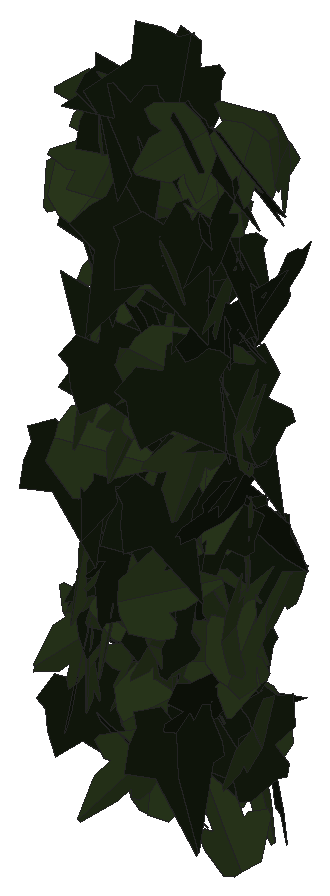
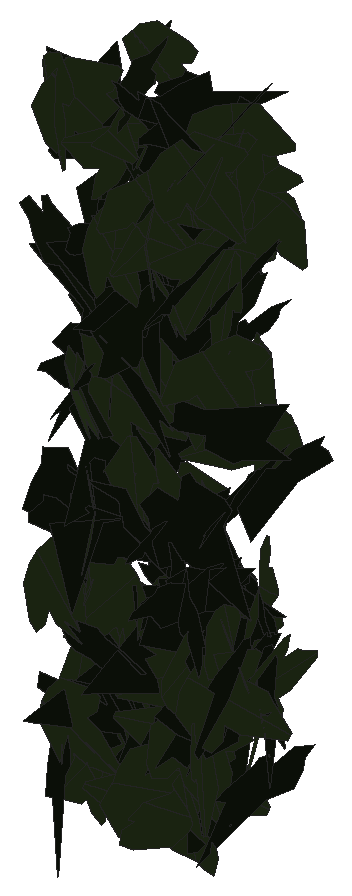
# SketchUp Ruby script. Lengths in inches.
U = 1.inch
M = Sketchup.active_model
def pt(a) = Geom::Point3d.new(a.map { |v| v * U })
def face(e, loops, mat)
  f = e.add_face(loops[0].map { |a| pt(a) })
  loops[1..].each { |l| e.add_face(l.map { |a| pt(a) }).erase! }
  f.material = f.back_material = mat if mat
  f
end
# faces: each face lists its corners as indices into pts; further lists are holes
def faces(e, pts, list, mat = nil) = list.each { |f| face(e, (f[0].is_a?(Array) ? f : [f]).map { |l| l.map { |i| pts[i] } }, mat) }
# xy, xz, yz: faces in a plane at the given z, y or x. An outline is a flat list of corners, or four numbers for a rectangle; further outlines are holes
def ring(l) = l.size == 4 ? [[l[0], l[1]], [l[2], l[1]], [l[2], l[3]], [l[0], l[3]]] : l.each_slice(2).to_a
def flat(e, list, mat, &to3) = list.each { |f| face(e, (f[0].is_a?(Array) ? f : [f]).map { |l| ring(l).map { |u, v| to3.(u, v) } }, mat) }
def xy(e, z, list, mat = nil) = flat(e, list, mat) { |x, y| [x, y, z] }
def xz(e, y, list, mat = nil) = flat(e, list, mat) { |x, z| [x, y, z] }
def yz(e, x, list, mat = nil) = flat(e, list, mat) { |y, z| [x, y, z] }
def lines(e, pts, list) = list.each { |a, b| e.add_line(pt(pts[a]), pt(pts[b])) }
# prism: a flat outline (further loops are holes) pulled along v
def prism(e, loops, v, mat = nil)
  f = face(e, loops, mat); d = Geom::Vector3d.new(v.map { |x| x * U })
  f.pushpull(f.normal.samedirection?(d) ? d.length : -d.length)
end
def box(e, o, s, mat = nil) = prism(e, [[o, [o[0] + s[0], o[1], o[2]], [o[0] + s[0], o[1] + s[1], o[2]], [o[0], o[1] + s[1], o[2]]]], [0, 0, s[2]], mat)
def at(x, y, z, deg = 0) = Geom::Transformation.translation(pt([x, y, z])) * Geom::Transformation.rotation(ORIGIN, Z_AXIS, deg.degrees)
def axes(o, x, y, z) = Geom::Transformation.new([*x, 0, *y, 0, *z, 0, *pt(o).to_a, 1])
def part(name) = M.definitions.add(name)
# library, detail: a bought-in or finely detailed component or shape, given as its bounding box
def library(name, o, s) = part(name).tap { |d| box(d.entities, o, s) }
def detail(e, o, s) = box(e.add_group.entities, o, s)
def put(e, d, t, mat = nil) = e.add_instance(d, t).tap { |i| i.material = mat if mat }
def group(e, t, mat = nil) = e.add_group.tap { |g| g.transformation = t; g.material = mat if mat }.entities
root = M.entities
M.materials.add("efeu1").color = [18, 25, 13]
M.materials.add("efeu2").color = [43, 57, 29]
c1 = part("ivyleaf_10")
p = [[0,0.5,-0.03],[-0.0625,2.02,-0.43],[-0.19,2.01,-0.46],[-0.54,1.05,-0.29],[-0.52,0.625,-0.18],[-0.83,0.76,-0.28],
  [-1.16,0.64,-0.33],[-1.15,0.33,-0.24],[-0.77,-0.39,0.02],[-0.3,-0.51,0.16],[0.04,-0.48,0.23],[-0.02,2.01,-0.4375],
  [-0.06,2.01,-0.43],[0.04,-0.49,0.23],[0.67,-0.49,0.14],[1.38,0.36,-0.2],[1.375,0.51,-0.24],[0.81,0.65,-0.19],
  [0.62,0.59,-0.15],[0.6,1.09,-0.28],[0.5,1.23,-0.31]]
faces(c1.entities,p,[[0,1,2,3,4,5,6,7,8,9,10],[11,12,0,13,14,15,16,17,18,19,20]],"efeu2")
c2 = part("ivyleaf_9")
p = [[1.54,2.16,1.25],[1.36,2.04,1.19],[-0.21,0.99,0.68],[-0.71,1.11,0.82],[-0.85,0.86,0.67],[-0.8,0.17,0.21],
  [-0.9,-0.01,0.1],[-0.67,-0.16,-0.02],[-0.08,-0.08,-0.05],[-0.03,-0.6,-0.4],[0.65,-0.88,-0.66],[0.83,-0.6,-0.49],
  [1.29,-0.42,-0.43],[1.8125,-0.07,-0.26],[1.21,0.44,0.15]]
faces(c2.entities,p,[[0,1,2,3,4,5,6,7,8,9,10,11,12,13,14]],"efeu1")
put(root,c1,axes([29.89,224.04,220.11],[0.30494,0.33422,-0.21286],[-0.15847,-0.14332,-0.45205],[-0.36318,0.34316,0.01852]))
put(root,c2,axes([30.2,223.7,218.97],[-0.43443,-0.21215,-0.12752],[-0.11485,-0.05543,0.48346],[-0.21927,0.44935,-0.00057]))
put(root,c2,axes([29.72,223.25,214.81],[0.17409,-0.32513,-0.33762],[-0.09037,0.33011,-0.3645],[0.45992,0.18793,0.05617]))
put(root,c1,axes([30.17,223.75,215.83],[-0.14395,-0.20317,0.43359],[-0.26964,-0.33975,-0.24872],[0.39569,-0.30543,-0.01176]))
put(root,c1,axes([30.0625,223.5,222.72],[-0.42816,-0.24629,0.07763],[-0.06228,-0.04739,-0.49384],[0.25061,-0.43255,0.0099]))
put(root,c1,axes([29.74,223.27,221.67],[-0.37195,-0.1587,-0.29405],[0.33105,-0.11527,-0.35653],[0.04537,-0.45992,0.19083]))
put(root,c2,axes([30.23,222.65,215.52],[-0.0639,0.00995,-0.4958],[-0.45594,0.19543,0.06269],[0.19503,0.46012,-0.01591]))
put(root,c1,axes([29.93,223.13,215.63],[-0.09985,0.02061,0.48949],[0.12986,-0.48058,0.04673],[0.4724,0.13646,0.09062]))
put(root,c2,axes([29.92,223.375,216.18],[0.18121,-0.23235,-0.40395],[-0.23512,0.32862,-0.2945],[0.40235,0.29668,0.00983]))
put(root,c1,axes([30.24,224.05,222.4375],[-0.32313,-0.19015,0.3308],[-0.26721,-0.19666,-0.37406],[0.27237,-0.41853,0.02548]))
put(root,c2,axes([29.8,223.66,221],[0.07578,-0.48888,0.07251],[0.01029,-0.07178,-0.49471],[0.49412,0.07648,-0.00082]))
put(root,c1,axes([30.12,223.52,220.9375],[-0.42226,0.2421,0.11439],[-0.10975,0.03835,-0.4863],[-0.24424,-0.43579,0.02076]))
put(root,c1,axes([30.2,223.26,221.92],[-0.36648,-0.26166,0.21732],[-0.11958,-0.19996,-0.4424],[0.31842,-0.37623,0.08398]))
put(root,c1,axes([30.02,223.53,222.41],[-0.09888,0.48227,-0.08741],[0.01674,-0.08579,-0.4923],[-0.48984,-0.10029,0.00082]))
put(root,c1,axes([29.9,223.25,215.4],[-0.07581,0.16469,-0.46597],[0.18358,-0.42831,-0.18125],[-0.45886,-0.19857,0.00447]))
put(root,c2,axes([29.94,222.88,218.26],[0.02806,-0.4767,-0.14821],[-0.01231,0.14774,-0.47752],[0.49906,0.03045,-0.00344]))
put(root,c1,axes([30.125,223.64,222.43],[0.39925,0.27288,-0.12703],[-0.12757,-0.03772,-0.48198],[-0.27262,0.41727,0.0395]))
put(root,c1,axes([29.95,223.07,221.35],[0.34715,0.17892,-0.3122],[0.23996,0.20816,0.38612],[0.26815,-0.41792,0.05866]))
put(root,c1,axes([30.04,223.04,216.86],[-0.08265,0.28216,-0.40442],[0.0715,-0.39887,-0.2929],[-0.48791,-0.10625,0.02558]))
put(root,c1,axes([30.22,223.29,216.4],[-0.02448,-0.49891,0.02214],[-0.00154,-0.02209,-0.49951],[0.4994,-0.02452,-0.00046]))
put(root,c2,axes([30.07,223.47,218.04],[-0.02876,-0.43143,0.25109],[-0.02001,-0.25031,-0.43237],[0.49877,-0.03492,-0.00287]))
put(root,c1,axes([30.26,223.72,215.18],[0.11648,-0.45418,-0.17365],[-0.03091,0.17128,-0.46873],[0.48526,0.11993,0.01182]))
put(root,c2,axes([29.9375,223.57,220.41],[0.27376,-0.3778,0.17979],[0.10296,-0.14742,-0.46655],[0.40553,0.29246,-0.00292]))
put(root,c2,axes([29.99,223.48,215.57],[0.45929,0.18219,-0.07657],[0.06581,0.04168,0.49389],[0.18635,-0.46376,0.01431]))
put(root,c2,axes([30.13,223.65,222.61],[0.02105,-0.4598,0.1953],[0.03429,-0.19368,-0.45969],[0.49838,0.03275,0.02337]))
put(root,c1,axes([30.53,223.625,215.15],[-0.41358,-0.18054,0.21531],[-0.19154,-0.09918,-0.45108],[0.20559,-0.45559,0.01288]))
put(root,c1,axes([30.43,222.5625,219.29],[0.07971,-0.30597,-0.38734],[-0.02744,0.389,-0.31293],[0.49284,0.07115,0.04522]))
put(root,c2,axes([30.66,223.61,217.9],[0.10002,0.06353,-0.48576],[-0.42356,-0.2379,-0.11833],[-0.24616,0.43516,0.00623]))
put(root,c2,axes([30.54,223.8,216.95],[-0.368,-0.27314,0.19992],[-0.1459,-0.13848,-0.45775],[0.30543,-0.39524,0.02222]))
put(root,c2,axes([30.5,223.26,216.61],[0.16095,0.42213,-0.21424],[-0.0791,-0.19912,-0.45177],[-0.46673,0.17931,0.00269]))
put(root,c1,axes([30.23,223.52,221],[0.27389,0.38408,0.16573],[0.10791,0.12652,-0.47154],[-0.40415,0.29407,-0.01359]))
put(root,c1,axes([30.3,223.21,216.28],[0.31118,-0.32028,0.22492],[0.15532,-0.16268,-0.44655],[0.35923,0.34778,-0.00175]))
put(root,c2,axes([30.65,223.94,222.8],[-0.25821,-0.14221,0.40386],[-0.31037,-0.26272,-0.29094],[0.29496,-0.40094,0.0474]))
put(root,c2,axes([30.24,223.9375,221.01],[0.08508,-0.49197,0.02695],[0.00315,-0.0268,-0.49927],[0.4927,0.08512,-0.00146]))
put(root,c2,axes([30.33,223.875,217.14],[-0.05947,-0.47854,-0.13215],[0.04546,0.12729,-0.48138],[0.49436,-0.06927,0.02837]))
put(root,c2,axes([30.34,222.86,216.44],[-0.18461,0.26258,0.38337],[0.18075,-0.33945,0.31954],[0.42808,0.25657,0.03041]))
put(root,c1,axes([30.21,222.61,218.5],[-0.08133,-0.16392,-0.46531],[0.44068,0.18787,-0.14321],[0.22179,-0.4334,0.11392]))
put(root,c2,axes([30.25,224,217.0625],[-0.08055,-0.05197,-0.49073],[0.49337,-0.01871,-0.079],[-0.01015,-0.49694,0.05429]))
put(root,c1,axes([30.54,223.78,215.84],[-0.08313,0.21512,0.44364],[0.12017,-0.42749,0.2298],[0.47817,0.14483,0.01937]))
put(root,c2,axes([30.53,223.21,222.78],[-0.27718,-0.19558,-0.36731],[0.28707,0.22965,-0.3389],[0.30127,-0.39876,-0.01502]))
put(root,c1,axes([30.8,223.1,214.29],[-0.06879,-0.28666,0.40385],[-0.07049,-0.39791,-0.29445],[0.4902,-0.09745,0.01433]))
put(root,c2,axes([30.48,222.73,219.78],[0.21598,-0.36995,-0.25787],[-0.01763,0.27877,-0.4147],[0.4506,0.18823,0.10737]))
put(root,c1,axes([30.66,223.46,213.625],[0.49282,-0.07666,0.03545],[-0.03493,0.00613,0.49874],[-0.0769,-0.49405,0.00069]))
put(root,c1,axes([30.4,223.13,216.37],[0.15115,0.11001,0.46374],[0.32998,0.32688,-0.18509],[-0.3439,0.362,0.02621]))
put(root,c2,axes([30.83,224.0625,222.99],[-0.47329,-0.04402,-0.1551],[0.15547,0.00269,-0.47521],[0.04267,-0.49805,0.01115]))
put(root,c2,axes([30.39,223.23,214.28],[0.38006,-0.2456,0.21269],[0.18795,-0.10078,-0.45224],[0.26501,0.4237,0.01571]))
put(root,c2,axes([30.84,223.01,221.41],[-0.44867,-0.18317,-0.12305],[0.11194,0.05137,-0.48459],[0.19017,-0.46239,-0.00509]))
put(root,c2,axes([30.51,223.84,222.24],[0.25739,-0.42631,0.04479],[0.03179,-0.03311,-0.49789],[0.42748,0.25915,0.01006]))
put(root,c1,axes([30.84,223.99,221.89],[0.31471,0.30907,-0.23544],[-0.18179,-0.15065,-0.44075],[-0.34338,0.36302,0.01755]))
put(root,c1,axes([30.82,223.01,219.03],[0.04732,-0.46484,0.17801],[0.02363,-0.17651,-0.46721],[0.49719,0.05263,0.00526]))
put(root,c1,axes([30.53,223.57,215.97],[-0.29124,-0.01699,-0.40607],[0.40465,0.03448,-0.29166],[0.03792,-0.49852,-0.00634]))
put(root,c1,axes([31.01,224.02,214.52],[0.14227,0.15908,-0.45217],[-0.30372,-0.33498,-0.21341],[-0.37083,0.33538,0.00132]))
put(root,c1,axes([30.75,223.49,221.46],[-0.17837,-0.23153,-0.40568],[0.23499,0.33082,-0.29213],[0.40368,-0.29488,-0.0092]))
put(root,c1,axes([30.66,224.15,221.32],[0.11035,-0.18585,0.45087],[0.37075,-0.26834,-0.20135],[0.31681,0.37876,0.07858]))
put(root,c2,axes([30.78,223.47,215.375],[0.49105,-0.02484,-0.09086],[-0.09076,0.00414,-0.49168],[0.02518,0.49937,-0.00044]))
put(root,c1,axes([30.76,223.65,214.11],[-0.08705,-0.20897,0.44582],[0.22209,0.38739,0.22495],[-0.43943,0.23719,0.02538]))
put(root,c1,axes([30.89,223.67,220.59],[0.38177,-0.29913,0.12153],[0.09571,-0.07489,-0.48501],[0.30837,0.39359,0.00008]))
put(root,c1,axes([30.72,223.18,214.86],[0.11144,0.11115,-0.47458],[0.37088,0.29655,0.15654],[0.31627,-0.38692,-0.01635]))
put(root,c2,axes([30.65,223.55,220.48],[0.04176,-0.0259,-0.49758],[0.32679,0.37835,0.00773],[0.37611,-0.32586,0.04852]))
put(root,c2,axes([30.875,223.32,217.5],[-0.0114,-0.49174,-0.08981],[0.0088,0.08962,-0.49182],[0.49979,-0.01279,0.00661]))
put(root,c1,axes([30.69,222.99,220.98],[-0.17936,0.00028,-0.46672],[0.46478,-0.04548,-0.17864],[-0.04255,-0.49793,0.01605]))
put(root,c2,axes([30.94,223.2,215.93],[0.18063,0.26247,0.38533],[0.22897,0.31004,-0.31851],[-0.40613,0.29153,-0.00819]))
put(root,c1,axes([31.22,222.99,216.02],[-0.25185,0.42434,-0.0807],[-0.05819,0.05923,0.49306],[0.428,0.25774,0.01955]))
put(root,c1,axes([31.24,223.74,220.98],[0.03432,0.13573,-0.48],[-0.24374,-0.41522,-0.13484],[-0.43522,0.24325,0.03766]))
put(root,c2,axes([31.15,223.98,219.59],[-0.42999,0.01132,-0.25491],[0.25478,-0.00828,-0.43014],[-0.01396,-0.4998,0.00135]))
put(root,c1,axes([30.76,223.47,217.74],[0.21706,-0.02585,0.44969],[0.44805,-0.03883,-0.2185],[0.04622,0.49782,0.00631]))
put(root,c2,axes([31.57,223.38,220.82],[-0.43819,-0.1224,-0.20739],[-0.20076,-0.05216,0.45495],[-0.133,0.48197,-0.00343]))
put(root,c1,axes([30.83,222.78,219.42],[0.14331,-0.00351,0.47901],[0.47419,0.07188,-0.14134],[-0.06787,0.49479,0.02393]))
put(root,c2,axes([31.46,223.42,220.51],[0.19956,0.0403,-0.45668],[-0.45107,-0.07174,-0.20344],[-0.08192,0.49318,0.00773]))
put(root,c1,axes([31.3125,223.33,221.17],[-0.18665,-0.46105,-0.05096],[0.01523,0.04881,-0.49738],[0.4636,-0.18722,-0.00418]))
put(root,c1,axes([31.32,224.08,221.2],[0.02926,-0.46126,0.19076],[0.01072,-0.19046,-0.46218],[0.49903,0.03113,-0.00126]))
put(root,c1,axes([31.34,222.95,216.21],[-0.00039,-0.48205,-0.13275],[0.00281,0.13275,-0.48205],[0.49999,-0.00112,0.00261]))
put(root,c1,axes([31.5,222.64,221.48],[-0.33951,0.23044,0.28571],[-0.25081,0.13854,-0.40976],[-0.26802,-0.42155,0.02152]))
put(root,c2,axes([30.94,223.98,220.15],[0.24837,-0.28166,0.33012],[0.2452,-0.22274,-0.37452],[0.35803,0.34793,0.02748]))
put(root,c1,axes([31.72,223.51,218.94],[-0.13255,0.04093,0.48037],[-0.46174,-0.15408,-0.11428],[0.13868,-0.4739,0.07864]))
put(root,c2,axes([31.26,222.78,216.06],[-0.31716,0.26131,0.28483],[0.20889,-0.19414,0.4107],[0.32523,0.37951,0.01398]))
put(root,c1,axes([31.39,223.4375,215.92],[0.0866,-0.49209,0.01854],[0.00315,-0.01827,-0.49966],[0.49243,0.08666,-0.00006]))
put(root,c1,axes([31.63,223.47,219.79],[-0.31514,-0.24581,0.30044],[-0.23809,-0.18325,-0.39967],[0.3066,-0.39496,-0.00155]))
put(root,c2,axes([31.27,223.15,214.78],[0.03534,-0.48218,-0.1275],[-0.02473,0.12597,-0.48324],[0.49814,0.04046,-0.01495]))
put(root,c1,axes([31.66,222.89,222.9],[0.34703,-0.10054,-0.34564],[-0.33693,0.07827,-0.36105],[0.12671,0.48349,-0.01342]))
put(root,c2,axes([31.32,222.6875,218.1875],[0.15646,-0.40352,-0.25037],[-0.09634,0.23116,-0.43276],[0.46501,0.18367,-0.00542]))
put(root,c1,axes([31.13,223.58,214.52],[0.29144,-0.01456,0.40601],[0.40619,0.02042,-0.29084],[-0.00812,0.49937,0.02373]))
put(root,c1,axes([31.22,222.69,219.95],[-0.25427,-0.09516,-0.41987],[0.3963,0.13879,-0.27145],[0.16821,-0.47083,0.00485]))
put(root,c2,axes([31.54,223.75,221.125],[-0.30949,-0.39216,0.02069],[-0.00913,-0.01915,-0.49955],[0.39259,-0.30959,0.00469]))
put(root,c1,axes([31.38,222.34,216.92],[-0.00569,-0.03702,0.4986],[0.13242,0.48071,0.0372],[-0.48211,0.13247,0.00434]))
put(root,c1,axes([31.5,223.32,217.46],[0.41846,0.27012,-0.04385],[0.0317,0.03174,0.49798],[0.27182,-0.41956,0.00944]))
put(root,c2,axes([31.8,223.39,217.34],[-0.48163,0.09346,-0.09642],[-0.09507,0.01621,0.49061],[0.09483,0.49092,0.00216]))
put(root,c2,axes([31.39,223.52,215],[-0.25404,-0.10025,-0.41882],[0.37881,0.17929,-0.27269],[0.20486,-0.45585,-0.01514]))
put(root,c2,axes([31.45,222.7,221.7],[-0.02126,-0.38988,-0.31232],[-0.00303,0.31269,-0.39015],[0.49954,-0.01469,-0.01566]))
put(root,c2,axes([31.78,223.86,215.99],[-0.49455,-0.02275,-0.06999],[0.06987,0.00415,-0.49508],[0.02311,-0.49946,-0.00093]))
put(root,c2,axes([31.42,223.24,222.84],[0.38704,-0.3037,-0.08925],[-0.05659,0.07231,-0.4915],[0.31144,0.39056,0.02161]))
put(root,c1,axes([31.72,222.95,218.8125],[-0.11001,-0.47229,0.12183],[0.00146,-0.12521,-0.48407],[0.48775,-0.10615,0.02893]))
put(root,c1,axes([32.01,223.26,215.92],[0.14773,0.02903,-0.4768],[-0.47665,0.04174,-0.14514],[0.03137,0.49741,0.04]))
put(root,c1,axes([31.59,223.27,221.89],[0.16278,0.11886,-0.45757],[0.21268,0.41379,0.18315],[0.42222,-0.25426,0.08416]))
put(root,c2,axes([31.48,223.11,215.15],[0.27574,0.18299,0.37481],[0.30887,0.21237,-0.33091],[-0.2803,0.41402,0.00407]))
put(root,c1,axes([31.55,223.5625,216.5625],[-0.38254,0.11989,-0.29881],[0.2878,-0.08072,-0.40082],[-0.14435,-0.47866,-0.00725]))
put(root,c1,axes([32.06,223.82,222.6],[-0.26128,-0.15436,0.39737],[-0.3406,-0.20469,-0.30346],[0.25636,-0.42927,0.00182]))
put(root,c2,axes([31.6,223.04,215],[-0.27011,-0.05004,-0.41777],[0.41618,0.04129,-0.27403],[0.06193,-0.49577,0.01935]))
put(root,c1,axes([32.09,223.89,214.94],[0.1812,-0.04702,-0.46363],[-0.42578,0.1855,-0.18521],[0.18942,0.46193,0.02718]))
put(root,c2,axes([31.54,222.62,219.84],[0.1191,-0.31214,-0.372],[0.13253,0.38938,-0.28429],[0.46717,-0.03089,0.17549]))
put(root,c2,axes([32,223.16,218.9375],[0.01516,-0.1557,0.4749],[-0.04412,0.47284,0.15644],[-0.49782,-0.04665,0.00059]))
put(root,c1,axes([31.92,223.29,220.92],[0.18148,-0.45955,-0.07667],[-0.01139,0.07788,-0.49377],[0.46576,0.18097,0.0178]))
put(root,c2,axes([32.05,223.08,221.93],[-0.42771,0.20962,-0.15205],[0.13751,-0.06492,-0.47631],[-0.21944,-0.44927,-0.00211]))
put(root,c2,axes([32.14,223.65,219.28],[-0.34105,-0.23158,0.28294],[-0.2417,-0.14753,-0.41209],[0.27435,-0.41786,-0.01131]))
put(root,c2,axes([31.92,222.88,218.04],[0.14546,0.39593,0.26847],[0.09226,0.25212,-0.42181],[-0.46939,0.17225,0.00029]))
put(root,c1,axes([31.75,223.84,217.53],[-0.14446,0.21543,-0.42746],[0.18242,-0.38803,-0.25721],[-0.44255,-0.23027,0.03352]))
put(root,c2,axes([31.76,223.16,220.02],[0.06268,-0.05626,0.49285],[0.36846,0.33789,-0.00829],[-0.33213,0.36423,0.08382]))
put(root,c2,axes([31.9,223.83,217.41],[-0.36934,-0.22641,-0.24965],[0.2066,0.14051,-0.43309],[0.26628,-0.42308,-0.01024]))
put(root,c2,axes([32.34,223.53,214.82],[-0.39161,0.07071,0.30273],[-0.30285,0.02312,-0.39717],[-0.07017,-0.49443,0.02472]))
put(root,c2,axes([32.17,223.24,218.69],[-0.39573,0.2903,-0.09552],[0.07494,-0.05933,-0.49078],[-0.29628,-0.40275,0.00345]))
put(root,c1,axes([31.97,223.52,222.6],[0.48787,-0.09863,-0.04749],[-0.04639,0.01018,-0.49774],[0.09915,0.49007,0.00078]))
put(root,c2,axes([32.06,223.64,217.76],[0.35264,0.10735,-0.33782],[-0.32128,-0.10454,-0.36858],[-0.14977,0.47702,-0.00475]))
put(root,c2,axes([31.7,223.48,221.34],[0.21904,-0.39023,0.22303],[0.09813,-0.2006,-0.44736],[0.43862,0.23975,-0.01129]))
put(root,c1,axes([31.97,223.79,219.1],[0.26843,-0.36327,0.21443],[0.12524,-0.17407,-0.45168],[0.40282,0.2962,-0.00245]))
put(root,c2,axes([31.875,223.55,219.1875],[0.21947,-0.42761,-0.13779],[-0.06429,0.12187,-0.48064],[0.44464,0.22869,-0.00149]))
put(root,c2,axes([32.28,223.6875,214.42],[0.17667,-0.02289,-0.46719],[-0.45803,0.09281,-0.17775],[0.09486,0.49078,0.01183]))
put(root,c1,axes([32.3,222.96,213.64],[0.38763,0.00828,0.31571],[-0.31562,-0.00776,0.38772],[0.01132,-0.49987,-0.00079]))
put(root,c1,axes([31.83,223.8,214.3],[0.30107,-0.12028,0.38064],[0.37152,-0.08999,-0.32229],[0.14604,0.4769,0.03518]))
put(root,c1,axes([32.1875,223.98,216.72],[-0.00417,-0.46157,0.19218],[0.00365,-0.19221,-0.46157],[0.49997,-0.00245,0.00497]))
put(root,c1,axes([32.34,222.82,216.55],[-0.04916,0.06767,0.49295],[-0.30775,0.38511,-0.08356],[-0.39099,-0.31163,0.00379]))
put(root,c2,axes([31.88,223.63,222.22],[0.09774,-0.25312,0.41997],[0.26508,-0.33299,-0.26239],[0.41253,0.27395,0.0691]))
put(root,c1,axes([32.41,222.95,219.24],[-0.04481,0.11736,0.48396],[-0.31032,0.37346,-0.11929],[-0.38948,-0.31105,0.03937]))
put(root,c2,axes([32.47,223.67,220.84],[-0.35494,0.35001,-0.03883],[0.02886,-0.02604,-0.49849],[-0.35097,-0.35611,-0.00172]))
put(root,c1,axes([32.36,223.71,222.63],[0.30135,-0.22664,-0.32836],[-0.17182,0.29766,-0.36314],[0.36009,0.33171,0.10152]))
put(root,c1,axes([32.24,222.96,216.07],[0.09391,0.31108,-0.38001],[0.05393,0.37803,0.32278],[0.48813,-0.10161,0.03744]))
put(root,c1,axes([32.33,223.23,215.08],[0.00582,-0.39691,-0.30403],[-0.01269,0.30383,-0.39689],[0.49981,0.01234,-0.00653]))
